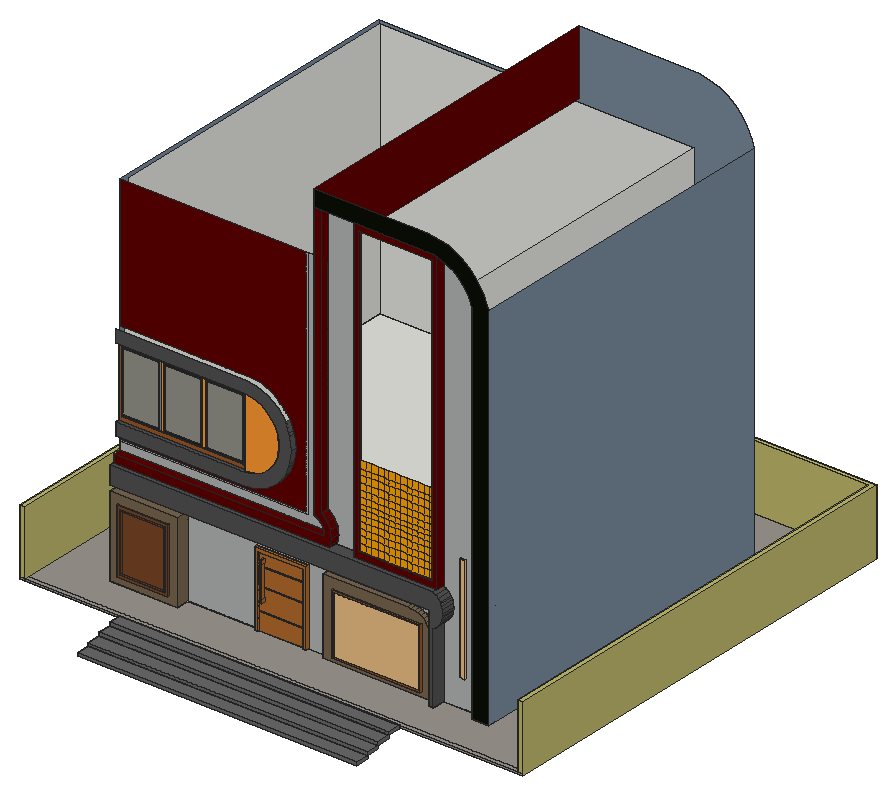
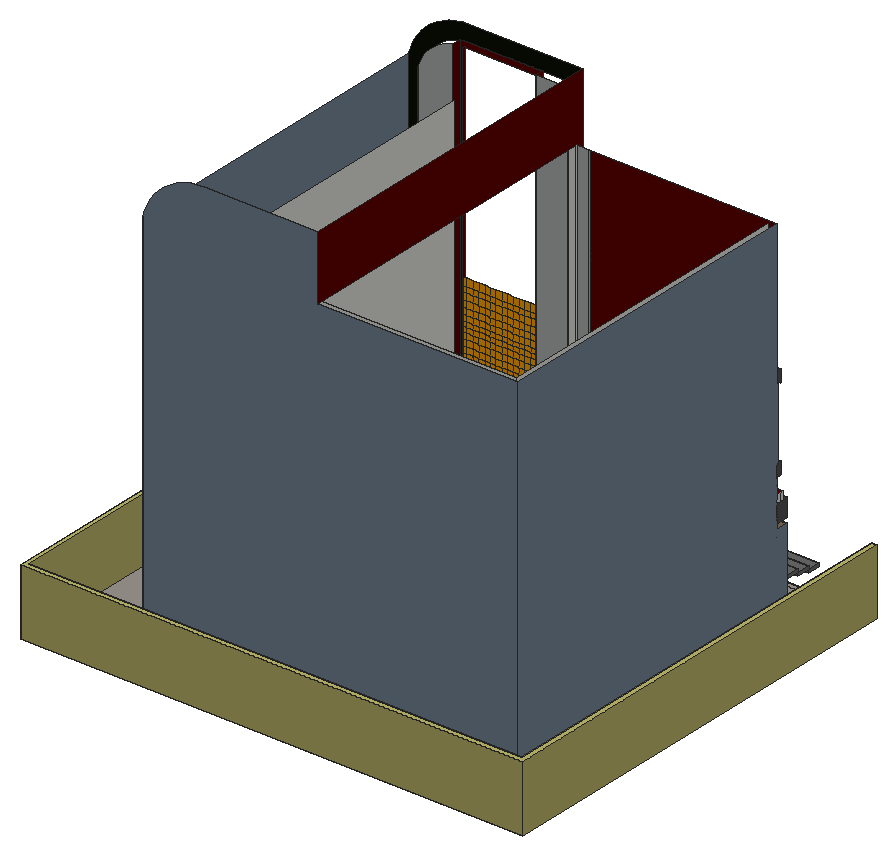
# SketchUp Ruby script. Lengths in inches.
U = 1.inch
M = Sketchup.active_model
def pt(a) = Geom::Point3d.new(a.map { |v| v * U })
def face(e, loops, mat)
  f = e.add_face(loops[0].map { |a| pt(a) })
  loops[1..].each { |l| e.add_face(l.map { |a| pt(a) }).erase! }
  f.material = f.back_material = mat if mat
  f
end
# faces: each face lists its corners as indices into pts; further lists are holes
def faces(e, pts, list, mat = nil) = list.each { |f| face(e, (f[0].is_a?(Array) ? f : [f]).map { |l| l.map { |i| pts[i] } }, mat) }
# xy, xz, yz: faces in a plane at the given z, y or x. An outline is a flat list of corners, or four numbers for a rectangle; further outlines are holes
def ring(l) = l.size == 4 ? [[l[0], l[1]], [l[2], l[1]], [l[2], l[3]], [l[0], l[3]]] : l.each_slice(2).to_a
def flat(e, list, mat, &to3) = list.each { |f| face(e, (f[0].is_a?(Array) ? f : [f]).map { |l| ring(l).map { |u, v| to3.(u, v) } }, mat) }
def xy(e, z, list, mat = nil) = flat(e, list, mat) { |x, y| [x, y, z] }
def xz(e, y, list, mat = nil) = flat(e, list, mat) { |x, z| [x, y, z] }
def yz(e, x, list, mat = nil) = flat(e, list, mat) { |y, z| [x, y, z] }
def lines(e, pts, list) = list.each { |a, b| e.add_line(pt(pts[a]), pt(pts[b])) }
# prism: a flat outline (further loops are holes) pulled along v
def prism(e, loops, v, mat = nil)
  f = face(e, loops, mat); d = Geom::Vector3d.new(v.map { |x| x * U })
  f.pushpull(f.normal.samedirection?(d) ? d.length : -d.length)
end
def box(e, o, s, mat = nil) = prism(e, [[o, [o[0] + s[0], o[1], o[2]], [o[0] + s[0], o[1] + s[1], o[2]], [o[0], o[1] + s[1], o[2]]]], [0, 0, s[2]], mat)
def at(x, y, z, deg = 0) = Geom::Transformation.translation(pt([x, y, z])) * Geom::Transformation.rotation(ORIGIN, Z_AXIS, deg.degrees)
def axes(o, x, y, z) = Geom::Transformation.new([*x, 0, *y, 0, *z, 0, *pt(o).to_a, 1])
def part(name) = M.definitions.add(name)
# library, detail: a bought-in or finely detailed component or shape, given as its bounding box
def library(name, o, s) = part(name).tap { |d| box(d.entities, o, s) }
def detail(e, o, s) = box(e.add_group.entities, o, s)
def put(e, d, t, mat = nil) = e.add_instance(d, t).tap { |i| i.material = mat if mat }
def group(e, t, mat = nil) = e.add_group.tap { |g| g.transformation = t; g.material = mat if mat }.entities
root = M.entities
M.materials.add("[0021_DarkRed]").color = [96, 0, 0]
M.materials.add("[0035_Tan]").color = [119, 102, 79]
M.materials.add("[0038_Orange]").color = [255, 165, 0]
M.materials.add("[0057_DarkKhaki]").color = [189, 183, 107]
M.materials.add("[0059_DarkOliveGreen]").color = [12, 15, 6]
M.materials.add("[0110_LightSlateGray]").color = [119, 136, 153]
M.materials.add("[0134_DimGray]").color = [105, 105, 105]
M.materials.add("[0135_DarkGray]").color = [81, 81, 81]
M.materials.add("[Blacktop Old 02]").color = [178, 181, 181]
M.materials.add("[Color C04]").color = [255, 153, 50]
M.materials.add("[Color M08]").color = [30, 30, 30]
M.materials.add("[Granite Tile]").color = [155, 148, 143]
M.materials.add("[Wood Bamboo]").color = [177, 105, 43]
M.materials.add("[Wood Cherry Original]").color = [152, 86, 42]
M.materials.add("[Wood Veneer 01]").color = [120, 70, 37]
M.materials.add("[Wood Veneer 01]1").color = [120, 70, 37]
M.materials.add("z1").color = [147, 146, 137]
c1 = library("FRAME",[0,-1.78,0],[32.34,1.78,45.93])
c2 = part("Untitled (3)")
g1 = group(c2.entities,at(46.82,21.85,47.25),"[Wood Veneer 01]1")
xy(g1,0,[[0,-0.375,19.95,0]])
xy(g1,0.5,[[0.5,-0.375,19.45,-0.25]])
xy(g1,25.5,[[0.5,-0.375,19.45,-0.25]])
xy(g1,26,[[0,-0.375,19.95,0]])
xz(g1,-0.375,[[[0,0,19.95,26],[0.5,0.5,19.45,25.5]]])
xz(g1,-0.25,[[0.5,0.5,19.45,25.5]])
xz(g1,0,[[0,0,19.95,26]])
yz(g1,0,[[-0.375,0,0,26]])
yz(g1,0.5,[[-0.375,0.5,-0.25,25.5]])
yz(g1,19.45,[[-0.375,0.5,-0.25,25.5]])
yz(g1,19.95,[[-0.375,0,0,26]])
c3 = library("\# BE HERE BE THE",[0.52,0,0],[173.07,10.23,1])
c4 = part("Frame (1)")
xy(c4.entities,0.79,[[[363.37,474.07,642.98,866.08],[370.05,480.76,636.3,859.4]],[[674.5,474.08,954.93,866.68],[681.18,480.76,948.25,860]],[[52.54,474.99,332.66,865.85],[59.22,481.67,325.97,859.17]]],"[Color M08]")
xy(c4.entities,0.79,[[370.05,480.76,636.3,859.4],[681.18,480.76,948.25,860],[59.22,481.67,325.97,859.17]],"z1")
xz(c4.entities,474.07,[[363.37,0,642.98,0.79]],"z1")
xz(c4.entities,474.08,[[674.5,0,954.93,0.79]],"z1")
xz(c4.entities,474.99,[[52.54,0,332.66,0.79]],"z1")
xz(c4.entities,865.85,[[52.54,0,332.66,0.79]],"z1")
xz(c4.entities,866.08,[[363.37,0,642.98,0.79]],"z1")
xz(c4.entities,866.68,[[674.5,0,954.93,0.79]],"z1")
yz(c4.entities,52.54,[[474.99,0,865.85,0.79]],"z1")
yz(c4.entities,332.66,[[474.99,0,865.85,0.79]],"z1")
yz(c4.entities,363.37,[[474.07,0,866.08,0.79]],"z1")
yz(c4.entities,642.98,[[474.07,0,866.08,0.79]],"z1")
yz(c4.entities,674.5,[[474.08,0,866.68,0.79]],"z1")
yz(c4.entities,954.93,[[474.08,0,866.68,0.79]],"z1")
xy(root,0,[[[0,97.75,930.625,917.0625],[108.0625,169.1875,233.9375,169.1875,233.9375,193.1875,362.17,193.1875,362.17,187.1875,368.17,187.1875,368.17,190.1875,451.67,190.1875,451.67,187.1875,457.67,187.1875,457.67,193.1875,698.91,193.1875,698.91,169.1875,708.0625,169.1875,708.0625,193.1875,772.36,193.1875,772.36,178.1875,802.875,178.1875,802.875,793.1875,108.0625,793.1875]],[[108.0625,169.1875,108.0625,793.1875,802.875,793.1875,802.875,193.1875,708.0625,193.1875,708.0625,169.1875,698.91,169.1875,698.91,193.1875,233.9375,193.1875,233.9375,169.1875],[117.0625,202.1875,699.0625,784.1875]],[362.17,187.1875,368.17,193.1875],[451.67,187.1875,457.67,193.1875],[368.17,190.1875,451.67,193.1875],
  [117.0625,202.1875,699.0625,784.1875]])
xy(root,3,[[9,97.75,921.625,106.75],[[9,106.75,921.625,908.0625],[108.0625,169.1875,108.0625,793.1875,802.875,793.1875,802.875,178.1875,772.36,178.1875,772.36,193.1875,708.0625,193.1875,708.0625,169.1875,698.91,169.1875,698.91,193.1875,457.67,193.1875,457.67,187.1875,451.67,187.1875,451.67,190.1875,368.17,190.1875,368.17,187.1875,362.17,187.1875,362.17,193.1875,233.9375,193.1875,233.9375,169.1875]]],"[Granite Tile]")
xy(root,5.23,[[493.6,181.1875,698.91,193.1875]])
xy(root,13.25,[[512.66,178.1875,676.39,181.1875]],"[Wood Cherry Original]")
xy(root,16.14,[[124.2,166.1875,217.8,169.1875]])
xy(root,16.43,[[515.84,178.1875,673.21,181.1875]],"[Wood Cherry Original]")
xy(root,22.33,[[130.39,166.1875,211.61,169.1875]],"[Wood Veneer 01]")
xy(root,53.55,[[375.78,184.1875,378.91,190.1875]],"[Wood Bamboo]")
xy(root,60.55,[[375.78,184.1875,378.91,190.1875]],"[Wood Bamboo]")
xy(root,118.36,[[375.78,184.1875,378.91,190.1875]],"[Wood Bamboo]")
xy(root,123,[[0,97.75,9,97.75,9,908.0625,921.625,908.0625,921.625,97.75,930.625,97.75,930.625,917.0625,0,917.0625]],"[0057_DarkKhaki]")
xy(root,123.18,[[515.84,178.1875,673.21,181.1875]],"[Wood Cherry Original]")
xy(root,125.36,[[375.78,184.1875,378.91,190.1875]])
xy(root,126.35,[[512.66,178.1875,676.39,181.1875]],"[Wood Cherry Original]")
xy(root,129.61,[[130.39,166.1875,211.61,169.1875]])
xy(root,135.11,[[368.17,190.1875,451.67,193.1875]])
xy(root,135.11,[[368.17,187.1875,451.67,190.1875]],"[Wood Bamboo]")
xy(root,135.8,[[124.2,166.1875,217.8,169.1875]],"[Wood Veneer 01]")
xy(root,141.11,[[362.17,187.1875,457.67,193.1875]],"[Wood Bamboo]")
xy(root,144.79,[[493.6,181.1875,651.15,193.1875]],"[0035_Tan]")
xy(root,151.9375,[[108.0625,169.1875,233.9375,193.1875]],"[0035_Tan]")
xy(root,161.8125,[[108.0625,169.1875,698.91,193.1875]],"[0135_DarkGray]")
xy(root,180,[[117.0625,193.1875,699.0625,202.1875],[117.0625,202.1875,699.0625,784.1875]])
xy(root,195.3,[[108.0625,178.1875,445.87,184.1875],[445.87,178.1875,491.99,184.1875],[491.99,178.1875,493.05,184.1875],[493.05,178.1875,499.36,184.1875],[499.36,178.1875,499.61,184.1875],
  [499.61,178.1875,501.6875,184.1875],[501.6875,178.1875,509.3,184.1875],[554.01,178.1875,699.0625,193.1875],[699.0625,178.1875,707.96,193.1875],[108.0625,184.1875,445.87,193.1875],
  [445.87,184.1875,491.99,193.1875],[491.99,184.1875,493.05,193.1875],[493.05,184.1875,499.36,193.1875],[499.36,184.1875,499.61,193.1875],[499.61,184.1875,501.6875,193.1875],
  [501.6875,184.1875,509.3,193.1875],[493.05,193.1875,499.36,194.875],[499.61,193.1875,509.3,194.875]])
xy(root,195.3,[[108.0625,169.1875,708.0625,169.1875,708.0625,193.1875,707.96,193.1875,707.96,178.1875,554.01,178.1875,554.01,193.1875,509.3,193.1875,509.3,178.1875,108.0625,178.1875]],"[0135_DarkGray]")
xy(root,207.09,[[563.08,178.1875,698.89,181.1875]],"[0021_DarkRed]")
xy(root,210.14,[[499.36,193.1875,499.61,194.875]])
xy(root,210.14,[[108.0625,178.1875,498.31,193.1875]],"[0021_DarkRed]")
xy(root,238.18,[[108.0625,183.5625,347.17,193.1875]],"[0135_DarkGray]")
xy(root,261.3125,[[108.0625,183.5625,345.65,190.1875]],"[0135_DarkGray]")
xy(root,267.69,[[114.44,190.1875,339.27,193.1875]],"[Wood Cherry Original]")
xz(root,97.75,[[0,3,9,123],[921.625,3,930.625,123]],"[0057_DarkKhaki]")
xz(root,97.75,[[0,0,930.625,3]],"[Granite Tile]")
xz(root,166.1875,[[[124.2,16.14,217.8,135.8],[130.39,22.33,211.61,129.61]]],"[Wood Veneer 01]")
xz(root,169.1875,[[108.0625,0,233.9375,3],[698.91,0,708.0625,3],[130.39,22.33,211.61,129.61]])
xz(root,169.1875,[[[108.0625,3,233.9375,151.9375],[124.2,16.14,217.8,135.8]]],"[0035_Tan]")
xz(root,169.1875,[[698.91,3,708.0625,3,708.0625,134.58,713.28,137.95,717.8,142.2,721.49,147.2,724.21,152.78,725.875,158.76,726.15,161.8125,726.4375,164.94,725.875,171.125,724.21,177.1,722.8,180,721.49,182.69,717.8,187.68,713.28,191.94,708.0625,195.3,108.0625,195.3,108.0625,161.8125,698.91,161.8125]],"[0135_DarkGray]")
xz(root,178.1875,[[772.36,0,802.875,3]])
xz(root,178.1875,[[108.0625,195.3,509.3,195.3,510.74,198.02,513.1,211.4,511.23,224.85,505.3125,237.08,495.92,246.89,493.5,248.19,493.5,749.49,479.14,749.49,479.14,239.62,487.12,235.32,493.38,228.78,497.33,220.63,498.31,213.6,498.31,210.14,108.0625,210.14],[[554.01,195.3,707.96,195.3,707.96,747.32,698.89,748.85,698.51,748.91,688.0625,749.49,554.01,749.49],[563.08,207.09,698.89,739.49]]],"[0021_DarkRed]")
xz(root,178.1875,[[772.36,3,802.875,3,802.875,690.57,799.09,703.01,793.95,714.96,787.52,726.26,780.13,736.43,779.87,736.78,771.11,746.39,761.34,754.97,750.68,762.42,739.26,768.65,727.23,773.57,714.72,777.125,701.89,779.28,688.91,780,479.14,780,479.14,749.49,688.0625,749.49,698.51,748.91,698.89,748.85,707.96,747.32,708,747.32,717.25,744.68,726.15,741.04,734.21,736.65,734.59,736.44,742.48,730.93,749.7,724.59,756.18,717.48,761.83,709.7,766.59,701.34,770.39,692.5,772.36,686.03]],"[0059_DarkOliveGreen]")
xz(root,178.1875,[[[512.66,13.25,676.39,126.35],[515.84,16.43,673.21,123.18]]],"[Wood Cherry Original]")
xz(root,181.1875,[[515.84,16.43,673.21,123.18]])
xz(root,181.1875,[[[493.6,5.23,698.91,5.23,698.91,97.03,698.5,103.27,697.28,109.39,695.27,115.31,692.51,120.91,689.04,126.11,684.92,130.8,680.22,134.92,675.03,138.39,669.43,141.16,663.51,143.16,657.39,144.38,651.15,144.79,493.6,144.79],[512.66,13.25,676.39,126.35]]],"[0035_Tan]")
xz(root,181.1875,[[563.08,207.09,573.89,220.18],[573.89,207.09,584.58,220.18],[584.58,207.09,595.27,220.18],[595.27,207.09,605.96,220.18],[605.96,207.09,616.64,220.18],
  [616.64,207.09,627.33,220.18],[627.33,207.09,638.02,220.18],[638.02,207.09,648.71,220.18],[648.71,207.09,659.39,220.18],[659.39,207.09,670.08,220.18],
  [670.08,207.09,680.77,220.18],[680.77,207.09,691.46,220.18],[691.46,207.09,698.89,220.18],[563.08,220.18,573.89,233.27],[573.89,220.18,584.58,233.27],
  [584.58,220.18,595.27,233.27],[595.27,220.18,605.96,233.27],[605.96,220.18,616.64,233.27],[616.64,220.18,627.33,233.27],[627.33,220.18,638.02,233.27],
  [638.02,220.18,648.71,233.27],[648.71,220.18,659.39,233.27],[659.39,220.18,670.08,233.27],[670.08,220.18,680.77,233.27],[680.77,220.18,691.46,233.27],
  [691.46,220.18,698.89,233.27],[563.08,233.27,573.89,244.83],[573.89,233.27,584.58,244.83],[584.58,233.27,595.27,244.83],[595.27,233.27,605.96,244.83],
  [605.96,233.27,616.64,244.83],[616.64,233.27,627.33,244.83],[627.33,233.27,638.02,244.83],[638.02,233.27,648.71,244.83],[648.71,233.27,659.39,244.83],
  [659.39,233.27,670.08,244.83],[670.08,233.27,680.77,244.83],[680.77,233.27,691.46,244.83],[691.46,233.27,698.89,244.83],[563.08,244.83,573.89,256.6875],
  [573.89,244.83,584.58,256.6875],[584.58,244.83,595.27,256.6875],[595.27,244.83,605.96,256.6875],[605.96,244.83,616.64,256.6875],[616.64,244.83,627.33,256.6875],
  [627.33,244.83,638.02,256.6875],[638.02,244.83,648.71,256.6875],[648.71,244.83,659.39,256.6875],[659.39,244.83,670.08,256.6875],[670.08,244.83,680.77,256.6875],
  [680.77,244.83,691.46,256.6875],[691.46,244.83,698.89,256.6875],[563.08,256.6875,573.89,267.83],[573.89,256.6875,584.58,267.83],[584.58,256.6875,595.27,267.83],
  [595.27,256.6875,605.96,267.83],[605.96,256.6875,616.64,267.83],[616.64,256.6875,627.33,267.83],[627.33,256.6875,638.02,267.83],[638.02,256.6875,648.71,267.83],
  [648.71,256.6875,659.39,267.83],[659.39,256.6875,670.08,267.83],[670.08,256.6875,680.77,267.83],[680.77,256.6875,691.46,267.83],[691.46,256.6875,698.89,267.83],
  [563.08,267.83,573.89,277.24],[573.89,267.83,584.58,277.24],[584.58,267.83,595.27,277.24],[595.27,267.83,605.96,277.24],[605.96,267.83,616.64,277.24],
  [616.64,267.83,627.33,277.24],[627.33,267.83,638.02,277.24],[638.02,267.83,648.71,277.24],[648.71,267.83,659.39,277.24],[659.39,267.83,670.08,277.24],
  [670.08,267.83,680.77,277.24],[680.77,267.83,691.46,277.24],[691.46,267.83,698.89,277.24],[563.08,277.24,573.89,286.02],[573.89,277.24,584.58,286.02],
  [584.58,277.24,595.27,286.02],[595.27,277.24,605.96,286.02],[605.96,277.24,616.64,286.02],[616.64,277.24,627.33,286.02],[627.33,277.24,638.02,286.02],
  [638.02,277.24,648.71,286.02],[648.71,277.24,659.39,286.02],[659.39,277.24,670.08,286.02],[670.08,277.24,680.77,286.02],[680.77,277.24,691.46,286.02],
  [691.46,277.24,698.89,286.02],[563.08,286.02,573.89,297.46],[573.89,286.02,584.58,297.46],[584.58,286.02,595.27,297.46],[595.27,286.02,605.96,297.46],
  [605.96,286.02,616.64,297.46],[616.64,286.02,627.33,297.46],[627.33,286.02,638.02,297.46],[638.02,286.02,648.71,297.46],[648.71,286.02,659.39,297.46],
  [659.39,286.02,670.08,297.46],[670.08,286.02,680.77,297.46],[680.77,286.02,691.46,297.46],[691.46,286.02,698.89,297.46],[563.08,297.46,573.89,309.06],
  [573.89,297.46,584.58,309.06],[584.58,297.46,595.27,309.06],[595.27,297.46,605.96,309.06],[605.96,297.46,616.64,309.06],[616.64,297.46,627.33,309.06],
  [627.33,297.46,638.02,309.06],[638.02,297.46,648.71,309.06],[648.71,297.46,659.39,309.06],[659.39,297.46,670.08,309.06],[670.08,297.46,680.77,309.06],
  [680.77,297.46,691.46,309.06],[691.46,297.46,698.89,309.06],[563.08,309.06,573.89,321.33],[573.89,309.06,584.58,321.33],[584.58,309.06,595.27,321.33],
  [595.27,309.06,605.96,321.33],[605.96,309.06,616.64,321.33],[616.64,309.06,627.33,321.33],[627.33,309.06,638.02,321.33],[638.02,309.06,648.71,321.33],
  [648.71,309.06,659.39,321.33],[659.39,309.06,670.08,321.33],[670.08,309.06,680.77,321.33],[680.77,309.06,691.46,321.33],[691.46,309.06,698.89,321.33],
  [563.08,321.33,573.89,334.34],[573.89,321.33,584.58,334.34],[584.58,321.33,595.27,334.34],[595.27,321.33,605.96,334.34],[605.96,321.33,616.64,334.34],
  [616.64,321.33,627.33,334.34],[627.33,321.33,638.02,334.34],[638.02,321.33,648.71,334.34],[648.71,321.33,659.39,334.34],[659.39,321.33,670.08,334.34],
  [670.08,321.33,680.77,334.34],[680.77,321.33,691.46,334.34],[691.46,321.33,698.89,334.34],[563.08,334.34,573.89,344.6],[573.89,334.34,584.58,344.6],
  [584.58,334.34,595.27,344.6],[595.27,334.34,605.96,344.6],[605.96,334.34,616.64,344.6],[616.64,334.34,627.33,344.6],[627.33,334.34,638.02,344.6],
  [638.02,334.34,648.71,344.6],[648.71,334.34,659.39,344.6],[659.39,334.34,670.08,344.6],[670.08,334.34,680.77,344.6],[680.77,334.34,691.46,344.6],
  [691.46,334.34,698.89,344.6],[563.08,344.6,573.89,358.98],[573.89,344.6,584.58,358.98],[584.58,344.6,595.27,358.98],[595.27,344.6,605.96,358.98],
  [605.96,344.6,616.64,358.98],[616.64,344.6,627.33,358.98],[627.33,344.6,638.02,358.98],[638.02,344.6,648.71,358.98],[648.71,344.6,659.39,358.98],
  [659.39,344.6,670.08,358.98],[670.08,344.6,680.77,358.98],[680.77,344.6,691.46,358.98],[691.46,344.6,698.89,358.98]],"[0038_Orange]")
xz(root,183.5625,[[108.0625,238.18,347.17,238.18,368.59,241,389.97,249.86,408.33,263.95,422.42,282.3,429.18,298.64,431.27,303.68,434.29,326.625,431.27,349.57,429.18,354.61,422.42,370.95,408.33,389.31,389.97,403.39,368.59,412.25,347.17,415.07,108.0625,415.07,108.0625,391.9375,345.65,391.9375,362.55,389.71,378.31,383.1875,391.83,372.81,402.21,359.28,407.8125,345.76,408.74,343.53,410.96,326.625,408.74,309.72,407.8125,307.49,402.21,293.97,391.83,280.44,378.31,270.0625,362.55,263.54,345.65,261.3125,108.0625,261.3125]],"[0135_DarkGray]")
xz(root,184.1875,[[375.78,53.55,378.91,60.55],[375.78,60.55,378.91,118.36],[375.78,118.36,378.91,125.36]],"[Wood Bamboo]")
xz(root,186.75,[[345.65,261.3125,362.55,263.54,378.31,270.0625,391.83,280.44,402.21,293.97,407.8125,307.49,408.74,309.72,410.96,326.625,408.74,343.53,407.8125,345.76,402.21,359.28,391.83,372.81,378.31,383.1875,362.55,389.71,345.65,391.9375]],"[Color C04]")
xz(root,187.1875,[[362.17,0,368.17,3],[451.67,0,457.67,3]])
xz(root,187.1875,[[362.17,3,368.17,3,368.17,135.11,451.67,135.11,451.67,3,457.67,3,457.67,141.11,362.17,141.11]],"[Wood Bamboo]")
xz(root,190.1875,[[368.17,0,451.67,3],[368.17,34.66,451.67,36.38],[368.17,76.35,451.67,78.07],[368.17,110.41,451.67,112.13]])
xz(root,190.1875,[[368.17,3,451.67,34.66],[[368.17,36.38,451.67,76.35],[375.78,53.55,378.91,60.55]],[368.17,78.07,451.67,110.41],[[368.17,112.13,451.67,135.11],[375.78,118.36,378.91,125.36]]],"[Wood Bamboo]")
xz(root,190.1875,[[[108.0625,261.3125,345.65,391.9375],[114.44,267.69,339.27,385.5625]]],"[Wood Cherry Original]")
xz(root,193.1875,[[362.17,-6,457.67,0],[233.9375,0,362.17,3],[362.17,0,362.17,141.11,457.67,141.11,457.67,0,451.67,0,451.67,135.11,368.17,135.11,368.17,0],[457.67,0,698.91,3],[708.0625,0,772.36,3],
  [493.6,5.23,493.6,144.79,651.15,144.79,657.39,144.38,663.51,143.16,669.43,141.16,675.03,138.39,680.22,134.92,684.92,130.8,689.04,126.11,692.51,120.91,695.27,115.31,697.28,109.39,698.5,103.27,698.91,97.03,698.91,5.23],[108.0625,161.8125,108.0625,180,699.0625,180,699.0625,195.3,708.0625,195.3,713.28,191.94,717.8,187.68,721.49,182.69,722.8,180,724.21,177.1,725.875,171.125,726.4375,164.94,726.15,161.8125],[108.0625,180,117.0625,180.95],[117.0625,180,699.0625,180,699.0625,195.3,513.25,195.3,513.25,180.95,117.0625,180.95],[108.0625,180.95,117.0625,182.0625],
  [117.0625,180.95,445.87,195.3],[445.87,180.95,445.87,195.3,452.22,188.84,460.25,184.65,469.17,183.14,478.13,184.44,486.26,188.44,492.76,194.75,493.05,195.3,501.6875,195.3,501.6875,180.95],[501.6875,180.95,501.6875,195.3,509.3,195.3],[501.6875,180.95,509.3,195.3,513.25,195.3,513.25,180.95],[108.0625,182.0625,117.0625,195.3],
  [469.17,183.14,460.25,184.65,452.22,188.84,445.87,195.3,493.05,195.3,492.76,194.75,486.26,188.44,478.13,184.44],[117.0625,195.3,491.99,210.14],[499.61,195.3,509.3,195.3,510.74,198.02,513.1,211.4,511.23,224.85,505.3125,237.08,495.92,246.89,493.5,248.19,493.5,660,479.14,660,479.14,239.62,487.12,235.32,493.38,228.78,497.33,220.63,498.31,213.6,498.31,214.32,499.61,214.32],[491.99,195.3,493.05,195.3,497,202.75,498.31,210.14,491.99,210.14],[493.05,195.3,499.36,195.3,499.36,210.14,498.31,210.14,497,202.75],
  [499.36,195.3,499.61,210.14],[498.31,210.14,498.57,211.66,498.31,213.6,498.31,214.32,499.61,214.32,499.61,210.14],[498.31,210.14,498.57,211.66,498.31,213.6],[117.0625,238.18,347.17,238.18,355.86,239.33,117.0625,239.33],[117.0625,239.33,355.86,239.33,368.59,241,389.97,249.86,408.33,263.95,422.42,282.3,429.18,298.64,431.27,303.68,434.29,326.625,431.27,349.57,429.18,354.61,422.42,370.95,408.33,389.31,389.97,403.39,368.59,412.25,347.17,415.07,117.0625,415.07,117.0625,385.5625,339.27,385.5625,339.27,267.69,117.0625,267.69],
  [114.44,267.69,117.0625,385.5625]])
xz(root,193.1875,[[108.0625,227.8125,453.55,227.8125,453.55,660,108.0625,660,108.0625,415.07,347.17,415.07,368.59,412.25,389.97,403.39,408.33,389.31,422.42,370.95,429.18,354.61,431.27,349.57,434.29,326.625,431.27,303.68,429.18,298.64,422.42,282.3,408.33,263.95,389.97,249.86,368.59,241,355.86,239.33,347.17,238.18,108.0625,238.18]],"[0021_DarkRed]")
xz(root,193.1875,[[233.9375,3,362.17,3,362.17,141.11,457.67,141.11,457.67,3,698.91,3,698.91,5.23,493.6,5.23,493.6,144.79,651.15,144.79,657.39,144.38,663.51,143.16,669.43,141.16,675.03,138.39,680.22,134.92,684.92,130.8,689.04,126.11,692.51,120.91,695.27,115.31,697.28,109.39,698.5,103.27,698.91,97.03,698.91,161.8125,108.0625,161.8125,108.0625,151.9375,233.9375,151.9375],[708.0625,3,772.36,3,772.36,686.03,770.39,692.5,766.59,701.34,761.83,709.7,756.18,717.48,749.7,724.59,742.48,730.93,734.59,736.44,726.15,741.04,717.25,744.68,708,747.32,707.96,747.32,707.96,195.3,708.0625,195.3,713.28,191.94,717.8,187.68,721.49,182.69,722.8,180,724.21,177.1,725.875,171.125,726.4375,164.94,726.15,161.8125,725.875,158.76,724.21,152.78,721.49,147.2,717.8,142.2,713.28,137.95,708.0625,134.58],[509.3,195.3,554.01,195.3,554.01,749.49,493.5,749.49,493.5,248.19,495.92,246.89,505.3125,237.08,511.23,224.85,513.1,211.4,510.74,198.02],[108.0625,210.14,499.61,210.14,499.61,214.32,498.31,214.32,498.31,213.6,497.33,220.63,493.38,228.78,487.12,235.32,479.14,239.62,479.14,660,453.55,660,453.55,227.8125,108.0625,227.8125]],"[Blacktop Old 02]")
xz(root,193.1875,[[117.0625,267.69,339.27,385.5625]],"[Color C04]")
xz(root,194.875,[[493.05,195.3,497,202.75,498.31,210.14,498.31,213.6,497.33,220.63,493.38,228.78,487.12,235.32,479.14,239.62,479.14,660,493.5,660,493.5,248.19,495.92,246.89,505.3125,237.08,511.23,224.85,513.1,211.4,510.74,198.02,509.3,195.3,499.61,195.3,499.61,210.14,499.36,210.14,499.36,195.3]])
xz(root,202.1875,[[117.0625,0,699.0625,180]])
xz(root,212.8125,[[722.8,180,721.49,182.69,717.8,187.68,713.28,191.94,708.0625,195.3,772.36,195.3,772.36,180]])
xz(root,784.1875,[[117.0625,0,699.0625,180],[117.0625,180,699.0625,660]])
xz(root,793.1875,[[108.0625,0,802.875,3]])
xz(root,793.1875,[[108.0625,3,108.0625,660,479.14,660,479.14,780,688.91,780,701.89,779.28,714.72,777.125,727.23,773.57,739.26,768.65,750.68,762.42,761.34,754.97,771.11,746.39,779.87,736.78,780.13,736.43,787.52,726.26,793.95,714.96,799.09,703.01,802.875,690.57,802.875,3]],"[0110_LightSlateGray]")
xz(root,908.0625,[[9,3,921.625,123]],"[0057_DarkKhaki]")
xz(root,917.0625,[[0,0,930.625,123]],"[0057_DarkKhaki]")
yz(root,0,[[97.75,0,917.0625,123]],"[0057_DarkKhaki]")
yz(root,9,[[97.75,3,908.0625,123]],"[0057_DarkKhaki]")
yz(root,108.0625,[[169.1875,0,793.1875,3],[178.1875,195.3,184.1875,210.14],[184.1875,195.3,193.1875,210.14]])
yz(root,108.0625,[[169.1875,3,169.1875,151.9375,193.1875,151.9375,193.1875,261.3125,190.1875,261.3125,190.1875,391.9375,193.1875,392.57,193.1875,660,793.1875,660,793.1875,3]],"[0110_LightSlateGray]")
yz(root,108.0625,[[169.1875,161.8125,193.1875,195.3],[183.5625,238.18,193.1875,261.3125]],"[0135_DarkGray]")
yz(root,114.44,[[190.1875,267.69,193.1875,385.5625]],"[Wood Cherry Original]")
yz(root,117.0625,[[202.1875,0,784.1875,180],[202.1875,180,784.1875,660],[181.1875,180.95,193.1875,182.0625]])
yz(root,124.2,[[166.1875,16.14,169.1875,135.8]],"[Wood Veneer 01]")
yz(root,130.39,[[166.1875,22.33,169.1875,129.61]],"[Wood Veneer 01]")
yz(root,211.61,[[166.1875,22.33,169.1875,129.61]],"[Wood Veneer 01]")
yz(root,217.8,[[166.1875,16.14,169.1875,135.8]],"[Wood Veneer 01]")
yz(root,233.9375,[[169.1875,0,193.1875,3]])
yz(root,233.9375,[[169.1875,3,193.1875,151.9375]],"[0035_Tan]")
yz(root,339.27,[[190.1875,267.69,193.1875,385.5625]],"[Wood Cherry Original]")
yz(root,345.65,[[186.75,261.3125,190.1875,391.9375]])
yz(root,362.17,[[187.1875,0,193.1875,3]])
yz(root,362.17,[[187.1875,3,193.1875,141.11]],"[Wood Bamboo]")
yz(root,368.17,[[187.1875,0,190.1875,3],[190.1875,0,193.1875,135.11]])
yz(root,368.17,[[187.1875,3,190.1875,135.11]],"[Wood Bamboo]")
yz(root,375.78,[[184.1875,53.55,190.1875,60.55],[184.1875,60.55,187.1875,118.36],[184.1875,118.36,190.1875,125.36]],"[Wood Bamboo]")
yz(root,378.91,[[184.1875,53.55,190.1875,60.55],[184.1875,60.55,187.1875,118.36],[184.1875,118.36,190.1875,125.36]],"[Wood Bamboo]")
yz(root,451.67,[[187.1875,0,190.1875,3],[190.1875,0,193.1875,135.11]])
yz(root,451.67,[[187.1875,3,190.1875,135.11]],"[Wood Bamboo]")
yz(root,457.67,[[187.1875,0,193.1875,3]])
yz(root,457.67,[[187.1875,3,193.1875,141.11]],"[Wood Bamboo]")
yz(root,479.14,[[193.1875,239.62,194.875,660]])
yz(root,479.14,[[178.1875,239.62,178.1875,780,793.1875,780,793.1875,660,193.1875,660,193.1875,239.62]],"[0021_DarkRed]")
yz(root,493.5,[[193.1875,248.19,194.875,660]])
yz(root,493.5,[[178.1875,248.19,193.1875,749.49]],"[0021_DarkRed]")
yz(root,493.6,[[181.1875,5.23,193.1875,144.79]],"[0035_Tan]")
yz(root,498.31,[[193.1875,210.14,194.875,213.6]])
yz(root,498.31,[[178.1875,210.14,193.1875,213.6]],"[0021_DarkRed]")
yz(root,499.36,[[193.1875,195.3,194.875,210.14]])
yz(root,499.61,[[193.1875,195.3,194.875,210.14]])
yz(root,512.66,[[178.1875,13.25,181.1875,126.35]],"[Wood Cherry Original]")
yz(root,515.84,[[178.1875,16.43,181.1875,123.18]],"[Wood Cherry Original]")
yz(root,554.01,[[178.1875,195.3,193.1875,749.49]],"[0021_DarkRed]")
yz(root,563.08,[[178.1875,207.09,181.1875,739.49]],"[0021_DarkRed]")
yz(root,673.21,[[178.1875,16.43,181.1875,123.18]],"[Wood Cherry Original]")
yz(root,676.39,[[178.1875,13.25,181.1875,126.35]],"[Wood Cherry Original]")
yz(root,698.89,[[178.1875,207.09,181.1875,334.34],[178.1875,334.34,181.1875,739.49]],"[0021_DarkRed]")
yz(root,698.91,[[169.1875,0,193.1875,3],[169.1875,3,193.1875,5.23],[181.1875,5.23,193.1875,97.03]])
yz(root,698.91,[[169.1875,5.23,169.1875,161.8125,193.1875,161.8125,193.1875,97.03,181.1875,97.03,181.1875,5.23]],"[0135_DarkGray]")
yz(root,699.0625,[[202.1875,0,784.1875,180],[202.1875,180,784.1875,660]])
yz(root,707.96,[[178.1875,195.3,193.1875,747.32]],"[0021_DarkRed]")
yz(root,708.0625,[[169.1875,0,193.1875,3]])
yz(root,708.0625,[[169.1875,3,193.1875,134.58]],"[0135_DarkGray]")
yz(root,772.36,[[178.1875,0,193.1875,3],[193.1875,180,212.8125,195.3]])
yz(root,772.36,[[178.1875,3,193.1875,686.03]],"[0059_DarkOliveGreen]")
yz(root,802.875,[[178.1875,0,193.1875,3],[193.1875,0,793.1875,3]])
yz(root,802.875,[[178.1875,3,793.1875,690.57]],"[0110_LightSlateGray]")
yz(root,921.625,[[97.75,3,908.0625,123]],"[0057_DarkKhaki]")
yz(root,930.625,[[97.75,0,917.0625,123]],"[0057_DarkKhaki]")
p = [[698.91,193.1875,97.03],[698.5,193.1875,103.27],[698.5,181.1875,103.27],[698.91,181.1875,97.03],[697.28,193.1875,109.39],[697.28,181.1875,109.39],
  [695.27,193.1875,115.31],[695.27,181.1875,115.31],[692.51,193.1875,120.91],[692.51,181.1875,120.91],[689.04,193.1875,126.11],[689.04,181.1875,126.11],
  [684.92,193.1875,130.8],[684.92,181.1875,130.8],[680.22,193.1875,134.92],[680.22,181.1875,134.92],[708.0625,193.1875,134.58],[713.28,193.1875,137.95],
  [713.28,169.1875,137.95],[708.0625,169.1875,134.58],[675.03,193.1875,138.39],[675.03,181.1875,138.39],[717.8,193.1875,142.2],[717.8,169.1875,142.2],
  [669.43,193.1875,141.16],[669.43,181.1875,141.16],[663.51,193.1875,143.16],[663.51,181.1875,143.16],[721.49,193.1875,147.2],[721.49,169.1875,147.2],
  [657.39,193.1875,144.38],[657.39,181.1875,144.38],[651.15,193.1875,144.79],[651.15,181.1875,144.79],[724.21,193.1875,152.78],[724.21,169.1875,152.78],
  [725.875,193.1875,158.76],[725.875,169.1875,158.76],[726.15,193.1875,161.8125],[726.15,169.1875,161.8125],[726.4375,193.1875,164.94],[726.4375,169.1875,164.94],
  [725.875,193.1875,171.125],[725.875,169.1875,171.125],[724.21,193.1875,177.1],[724.21,169.1875,177.1],[722.8,193.1875,180],[722.8,169.1875,180],
  [721.49,193.1875,182.69],[721.49,169.1875,182.69],[721.49,212.8125,182.69],[722.8,212.8125,180],[717.8,193.1875,187.68],[717.8,169.1875,187.68],
  [717.8,212.8125,187.68],[713.28,193.1875,191.94],[713.28,169.1875,191.94],[713.28,212.8125,191.94],[708.0625,193.1875,195.3],[708.0625,169.1875,195.3],
  [708.0625,212.8125,195.3],[510.74,193.1875,198.02],[510.74,178.1875,198.02],[509.3,178.1875,195.3],[509.3,184.1875,195.3],[509.3,193.1875,195.3],
  [493.05,194.875,195.3],[493.05,193.1875,195.3],[497,193.1875,202.75],[497,194.875,202.75],[510.74,194.875,198.02],[509.3,194.875,195.3],
  [513.1,193.1875,211.4],[513.1,178.1875,211.4],[513.1,194.875,211.4],[498.31,193.1875,210.14],[498.31,194.875,210.14],[511.23,193.1875,224.85],
  [511.23,178.1875,224.85],[511.23,194.875,224.85],[498.31,193.1875,213.6],[498.31,178.1875,213.6],[497.33,178.1875,220.63],[497.33,193.1875,220.63],
  [498.31,194.875,213.6],[497.33,194.875,220.63],[493.38,178.1875,228.78],[493.38,193.1875,228.78],[493.38,194.875,228.78],[505.3125,193.1875,237.08],
  [505.3125,178.1875,237.08],[505.3125,194.875,237.08],[487.12,178.1875,235.32],[487.12,193.1875,235.32],[487.12,194.875,235.32],[479.14,178.1875,239.62],
  [479.14,193.1875,239.62],[479.14,194.875,239.62],[495.92,193.1875,246.89],[495.92,178.1875,246.89],[495.92,194.875,246.89],[347.17,193.1875,238.18],
  [355.86,193.1875,239.33],[368.59,193.1875,241],[368.59,183.5625,241],[347.17,183.5625,238.18],[389.97,193.1875,249.86],[389.97,183.5625,249.86],
  [493.5,193.1875,248.19],[493.5,178.1875,248.19],[493.5,194.875,248.19],[408.33,193.1875,263.95],[408.33,183.5625,263.95],[362.55,183.5625,263.54],
  [362.55,186.75,263.54],[345.65,186.75,261.3125],[345.65,183.5625,261.3125],[378.31,183.5625,270.0625],[378.31,186.75,270.0625],[422.42,193.1875,282.3],
  [422.42,183.5625,282.3],[391.83,183.5625,280.44],[391.83,186.75,280.44],[402.21,183.5625,293.97],[402.21,186.75,293.97],[429.18,193.1875,298.64],
  [429.18,183.5625,298.64],[407.8125,183.5625,307.49],[407.8125,186.75,307.49],[431.27,193.1875,303.68],[431.27,183.5625,303.68],[434.29,193.1875,326.625],
  [434.29,183.5625,326.625],[408.74,183.5625,309.72],[408.74,186.75,309.72],[410.96,183.5625,326.625],[410.96,186.75,326.625],[408.74,183.5625,343.53],
  [408.74,186.75,343.53],[431.27,193.1875,349.57],[431.27,183.5625,349.57],[407.8125,183.5625,345.76],[407.8125,186.75,345.76],[402.21,183.5625,359.28],
  [402.21,186.75,359.28],[429.18,193.1875,354.61],[429.18,183.5625,354.61],[422.42,193.1875,370.95],[422.42,183.5625,370.95],[108.0625,193.1875,139.5],
  [233.9375,193.1875,139.5],[456.42,193.1875,660],[456.42,193.1875,224.97],[108.0625,193.1875,224.97],[499.61,193.1875,214.32],[499.61,184.1875,214.32],
  [499.36,184.1875,210.14],[499.36,193.1875,210.14],[498.31,193.1875,214.32],[498.31,184.1875,214.32],[698.91,193.1875,0],[698.91,193.1875,-1.08],
  [699.0625,193.1875,180],[699.0625,181.1875,180],[513.25,193.1875,180.95],[513.25,181.1875,180.95],[501.6875,193.1875,180.95],[501.6875,181.1875,180.95],
  [501.6875,181.1875,195.3],[772.36,193.1875,195.3],[802.875,193.1875,195.3]]
faces(root,p,[[0,1,2,3],[1,4,5,2],[4,6,7,5],[6,8,9,7],[8,10,11,9],[10,12,13,11],[12,14,15,13],[14,20,21,15],
  [20,24,25,21],[24,26,27,25],[26,30,31,27],[30,32,33,31]],"[0035_Tan]")
faces(root,p,[[16,17,18,19],[17,22,23,18],[22,28,29,23],[28,34,35,29],[34,36,37,35],[36,38,39,37],[38,40,41,39],[40,42,43,41],
  [42,44,45,43],[44,46,47,45],[46,48,49,47],[48,52,53,49],[52,55,56,53],[55,58,59,56],[101,102,103,104,105],[103,106,107,104],
  [106,111,112,107],[113,114,115,116],[117,118,114,113],[111,119,120,112],[121,122,118,117],[123,124,122,121],[119,125,126,120],[127,128,124,123],
  [125,129,130,126],[129,131,132,130],[133,134,128,127],[135,136,134,133],[137,138,136,135],[131,139,140,132],[141,142,138,137],[143,144,142,141],
  [139,145,146,140],[145,147,148,146]],"[0135_DarkGray]")
faces(root,p,[[46,48,50,51],[48,52,54,50],[52,55,57,54],[55,58,60,57],[66,67,68,69],[70,61,65,71],[74,72,61,70],[69,68,75,76],
  [79,77,72,74],[84,80,83,85],[85,83,87,88],[91,89,77,79],[88,87,93,94],[94,93,96,97],[100,98,89,91],[110,108,98,100]])
faces(root,p,[[61,62,63,64,65],[72,73,62,61],[77,78,73,72],[80,81,82,83],[83,82,86,87],[89,90,78,77],[87,86,92,93],[93,92,95,96],
  [98,99,90,89],[108,109,99,98]],"[0021_DarkRed]")
lines(root,p,[[149,150],[151,152],[153,152],[154,155],[156,157],[158,159],[160,161],[162,163],[164,165],[166,167],[167,168],[169,170]])
g2 = group(root,at(184.0625,0,-21),"[0134_DimGray]")
xy(g2,0,[[0,0,517.875,24.6875]])
xy(g2,6,[[0,0,517.875,24.6875],[0,24.6875,517.875,49.375]])
xy(g2,12,[[0,24.6875,517.875,49.375],[0,49.375,517.875,74.0625]])
xy(g2,18,[[0,49.375,517.875,74.0625],[0,74.0625,517.875,98.75]])
xy(g2,24,[[0,74.0625,517.875,98.75]])
xz(g2,0,[[0,0,517.875,6]])
xz(g2,24.6875,[[0,0,517.875,6],[0,6,517.875,12]])
xz(g2,49.375,[[0,6,517.875,12],[0,12,517.875,18]])
xz(g2,74.0625,[[0,12,517.875,18],[0,18,517.875,24]])
xz(g2,98.75,[[0,18,517.875,24]])
yz(g2,0,[[0,0,24.6875,6],[24.6875,6,49.375,12],[49.375,12,74.0625,18],[74.0625,18,98.75,24]])
yz(g2,517.875,[[0,0,24.6875,6],[24.6875,6,49.375,12],[49.375,12,74.0625,18],[74.0625,18,98.75,24]])
put(root,c1,axes([515.84,182.32,16.49],[4.86656,0,0],[0,2.32278,0],[0,0,2.32278]))
put(root,c2,axes([-64.62,76.59,-174.47],[4.16493,0,0],[0,4.16493,0],[0,0,4.16493]))
put(root,c3,axes([749.95,193.1875,55.1],[0,0,1.14],[-1,0,0],[0,-3.27,0]))
put(root,c4,axes([101.91,190.98,131.74],[0.24972,0,0],[0,0,0.29286],[0,-1,0]))
